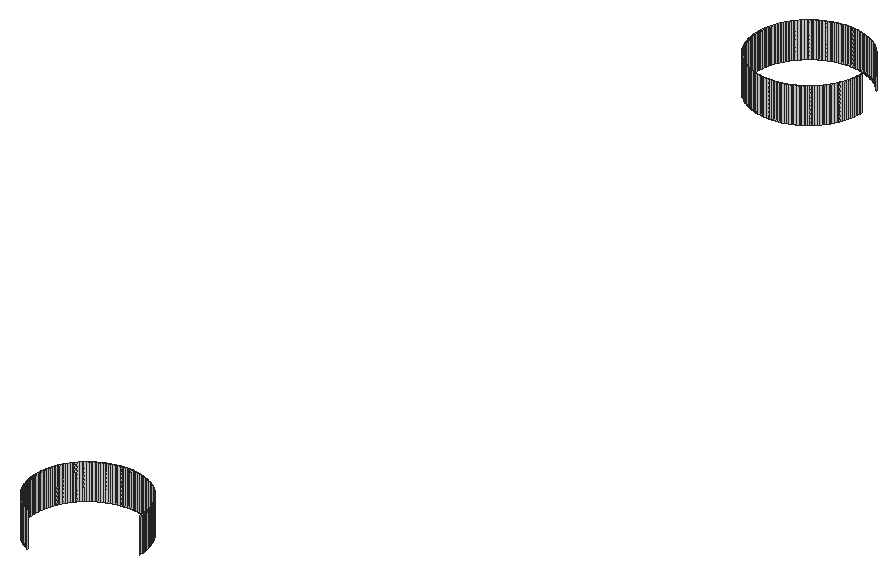
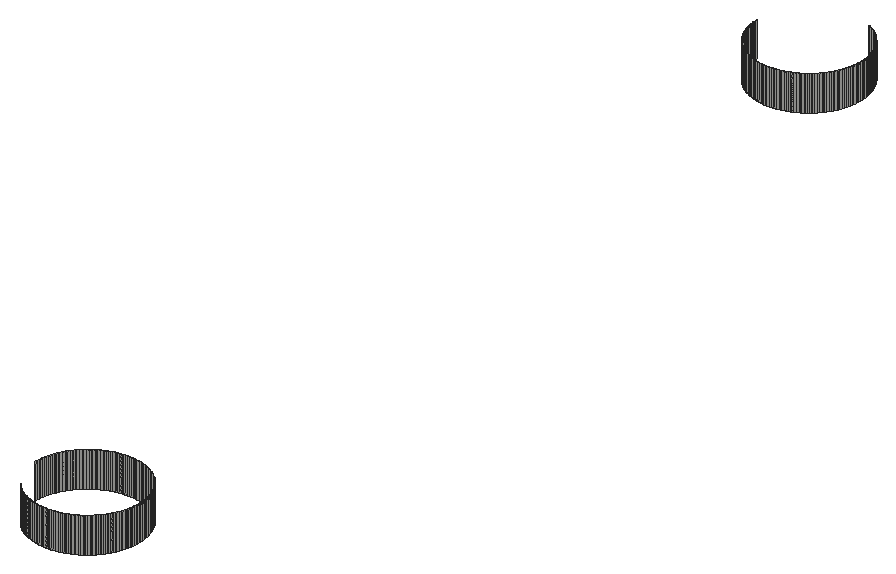
# SketchUp Ruby script. Lengths in inches.
U = 1.inch
M = Sketchup.active_model
def pt(a) = Geom::Point3d.new(a.map { |v| v * U })
def face(e, loops, mat)
  f = e.add_face(loops[0].map { |a| pt(a) })
  loops[1..].each { |l| e.add_face(l.map { |a| pt(a) }).erase! }
  f.material = f.back_material = mat if mat
  f
end
# faces: each face lists its corners as indices into pts; further lists are holes
def faces(e, pts, list, mat = nil) = list.each { |f| face(e, (f[0].is_a?(Array) ? f : [f]).map { |l| l.map { |i| pts[i] } }, mat) }
# xy, xz, yz: faces in a plane at the given z, y or x. An outline is a flat list of corners, or four numbers for a rectangle; further outlines are holes
def ring(l) = l.size == 4 ? [[l[0], l[1]], [l[2], l[1]], [l[2], l[3]], [l[0], l[3]]] : l.each_slice(2).to_a
def flat(e, list, mat, &to3) = list.each { |f| face(e, (f[0].is_a?(Array) ? f : [f]).map { |l| ring(l).map { |u, v| to3.(u, v) } }, mat) }
def xy(e, z, list, mat = nil) = flat(e, list, mat) { |x, y| [x, y, z] }
def xz(e, y, list, mat = nil) = flat(e, list, mat) { |x, z| [x, y, z] }
def yz(e, x, list, mat = nil) = flat(e, list, mat) { |y, z| [x, y, z] }
def lines(e, pts, list) = list.each { |a, b| e.add_line(pt(pts[a]), pt(pts[b])) }
# prism: a flat outline (further loops are holes) pulled along v
def prism(e, loops, v, mat = nil)
  f = face(e, loops, mat); d = Geom::Vector3d.new(v.map { |x| x * U })
  f.pushpull(f.normal.samedirection?(d) ? d.length : -d.length)
end
def box(e, o, s, mat = nil) = prism(e, [[o, [o[0] + s[0], o[1], o[2]], [o[0] + s[0], o[1] + s[1], o[2]], [o[0], o[1] + s[1], o[2]]]], [0, 0, s[2]], mat)
def at(x, y, z, deg = 0) = Geom::Transformation.translation(pt([x, y, z])) * Geom::Transformation.rotation(ORIGIN, Z_AXIS, deg.degrees)
def axes(o, x, y, z) = Geom::Transformation.new([*x, 0, *y, 0, *z, 0, *pt(o).to_a, 1])
def part(name) = M.definitions.add(name)
# library, detail: a bought-in or finely detailed component or shape, given as its bounding box
def library(name, o, s) = part(name).tap { |d| box(d.entities, o, s) }
def detail(e, o, s) = box(e.add_group.entities, o, s)
def put(e, d, t, mat = nil) = e.add_instance(d, t).tap { |i| i.material = mat if mat }
def group(e, t, mat = nil) = e.add_group.tap { |g| g.transformation = t; g.material = mat if mat }.entities
root = M.entities
xz(root,78.5,[[156.34,108,156.42,110],[156.42,108,156.5,110],[156.5,108,156.58,110],[156.58,108,156.66,110]])
xz(root,124,[[156.34,108,156.42,110],[156.42,108,156.5,110],[156.5,108,156.58,110],[156.58,108,156.66,110]])
xz(root,130,[[156.34,108,156.42,110],[156.42,108,156.5,110],[156.5,108,156.58,110],[156.58,108,156.66,110]])
yz(root,153.5,[[75.34,108,75.42,110],[75.42,108,75.5,110],[75.5,108,75.58,110],[75.58,108,75.66,110],[126.84,108,126.92,110],
  [126.92,108,127,110],[127,108,127.08,110],[127.08,108,127.16,110]])
yz(root,159.5,[[75.5,108,75.58,110],[75.58,108,75.66,110],[126.84,108,126.92,110],[126.92,108,127,110]])
p = [[155.21,72.79,108],[155.14,72.83,108],[155.14,72.83,110],[155.21,72.79,110],[155.07,72.86,108],[155.07,72.86,110],
  [155.28,72.76,108],[155.28,72.76,110],[155,72.9,108],[154.93,72.94,108],[154.93,72.94,110],[155,72.9,110],
  [154.87,72.98,108],[154.87,72.98,110],[154.8,73.03,108],[154.74,73.07,108],[154.74,73.07,110],[154.8,73.03,110],
  [154.67,73.12,108],[154.61,73.17,108],[154.61,73.17,110],[154.67,73.12,110],[154.55,73.22,108],[154.49,73.27,108],
  [154.49,73.27,110],[154.55,73.22,110],[154.43,73.32,108],[154.43,73.32,110],[154.38,73.38,108],[154.38,73.38,110],
  [154.32,73.43,108],[154.32,73.43,110],[154.27,73.49,108],[154.27,73.49,110],[154.22,73.55,108],[154.22,73.55,110],
  [154.17,73.61,108],[154.12,73.67,108],[154.12,73.67,110],[154.17,73.61,110],[154.07,73.74,108],[154.03,73.8,108],
  [154.03,73.8,110],[154.07,73.74,110],[153.98,73.87,108],[153.98,73.87,110],[153.94,73.93,108],[153.94,73.93,110],
  [153.9,74,108],[153.9,74,110],[153.86,74.07,108],[153.86,74.07,110],[153.83,74.14,108],[153.83,74.14,110],
  [153.79,74.21,108],[153.79,74.21,110],[153.76,74.28,108],[153.76,74.28,110],[153.73,74.35,108],[153.73,74.35,110],
  [153.7,74.42,108],[153.7,74.42,110],[153.67,74.5,108],[153.67,74.5,110],[153.65,74.57,108],[153.65,74.57,110],
  [153.625,74.65,108],[153.625,74.65,110],[153.6,74.72,108],[153.6,74.72,110],[153.58,74.8,108],[153.58,74.8,110],
  [153.57,74.875,108],[153.57,74.875,110],[153.55,74.95,108],[153.55,74.95,110],[153.54,75.03,108],[153.54,75.03,110],
  [153.53,75.11,108],[153.53,75.11,110],[153.52,75.1875,108],[153.52,75.1875,110],[153.51,75.26,108],[153.51,75.26,110],
  [153.5,75.34,108],[153.5,75.34,110],[153.5,75.66,108],[153.51,75.74,108],[153.51,75.74,110],[153.5,75.66,110],
  [153.52,75.8125,108],[153.52,75.8125,110],[159.48,75.8125,108],[159.49,75.74,108],[159.49,75.74,110],[159.48,75.8125,110],
  [159.5,75.66,108],[159.5,75.66,110],[153.53,75.89,108],[153.53,75.89,110],[159.47,75.89,108],[159.47,75.89,110],
  [153.54,75.97,108],[153.54,75.97,110],[159.46,75.97,108],[159.46,75.97,110],[153.55,76.05,108],[153.55,76.05,110],
  [153.57,76.125,108],[153.57,76.125,110],[159.43,76.125,108],[159.45,76.05,108],[159.45,76.05,110],[159.43,76.125,110],
  [153.58,76.2,108],[153.58,76.2,110],[159.42,76.2,108],[159.42,76.2,110],[153.6,76.28,108],[153.6,76.28,110],
  [159.4,76.28,108],[159.4,76.28,110],[153.625,76.35,108],[153.625,76.35,110],[159.375,76.35,108],[159.375,76.35,110],
  [153.65,76.43,108],[153.65,76.43,110],[153.67,76.5,108],[153.67,76.5,110],[159.33,76.5,108],[159.35,76.43,108],
  [159.35,76.43,110],[159.33,76.5,110],[153.7,76.58,108],[153.7,76.58,110],[159.3,76.58,108],[159.3,76.58,110],
  [153.73,76.65,108],[153.73,76.65,110],[153.76,76.72,108],[153.76,76.72,110],[159.24,76.72,108],[159.27,76.65,108],
  [159.27,76.65,110],[159.24,76.72,110],[153.79,76.79,108],[153.79,76.79,110],[159.21,76.79,108],[159.21,76.79,110],
  [153.83,76.86,108],[153.83,76.86,110],[159.17,76.86,108],[159.17,76.86,110],[153.86,76.93,108],[153.86,76.93,110],
  [153.9,77,108],[153.9,77,110],[159.1,77,108],[159.14,76.93,108],[159.14,76.93,110],[159.1,77,110],
  [153.94,77.07,108],[153.94,77.07,110],[159.06,77.07,108],[159.06,77.07,110],[153.98,77.13,108],[153.98,77.13,110],
  [154.03,77.2,108],[154.03,77.2,110],[158.97,77.2,108],[159.02,77.13,108],[159.02,77.13,110],[158.97,77.2,110],
  [154.07,77.26,108],[154.07,77.26,110],[158.93,77.26,108],[158.93,77.26,110],[154.12,77.33,108],[154.12,77.33,110],
  [154.17,77.39,108],[154.17,77.39,110],[158.83,77.39,108],[158.88,77.33,108],[158.88,77.33,110],[158.83,77.39,110],
  [154.22,77.45,108],[154.22,77.45,110],[154.27,77.51,108],[154.27,77.51,110],[158.73,77.51,108],[158.78,77.45,108],
  [158.78,77.45,110],[158.73,77.51,110],[154.32,77.57,108],[154.32,77.57,110],[158.68,77.57,108],[158.68,77.57,110],
  [154.38,77.62,108],[154.38,77.62,110],[154.43,77.68,108],[154.43,77.68,110],[158.57,77.68,108],[158.62,77.62,108],
  [158.62,77.62,110],[158.57,77.68,110],[154.49,77.73,108],[154.49,77.73,110],[154.55,77.78,108],[154.55,77.78,110],
  [158.45,77.78,108],[158.51,77.73,108],[158.51,77.73,110],[158.45,77.78,110],[154.61,77.83,108],[154.61,77.83,110],
  [154.67,77.88,108],[154.67,77.88,110],[158.33,77.88,108],[158.39,77.83,108],[158.39,77.83,110],[158.33,77.88,110],
  [154.74,77.93,108],[154.74,77.93,110],[154.8,77.97,108],[154.8,77.97,110],[158.2,77.97,108],[158.26,77.93,108],
  [158.26,77.93,110],[158.2,77.97,110],[154.87,78.02,108],[154.87,78.02,110],[154.93,78.06,108],[154.93,78.06,110],
  [158.07,78.06,108],[158.13,78.02,108],[158.13,78.02,110],[158.07,78.06,110],[155,78.1,108],[155,78.1,110],
  [155.07,78.14,108],[155.07,78.14,110],[155.14,78.17,108],[155.14,78.17,110],[157.86,78.17,108],[157.93,78.14,108],
  [157.93,78.14,110],[157.86,78.17,110],[158,78.1,108],[158,78.1,110],[155.21,78.21,108],[155.21,78.21,110],
  [155.28,78.24,108],[155.28,78.24,110],[155.35,78.27,108],[155.35,78.27,110],[157.65,78.27,108],[157.72,78.24,108],
  [157.72,78.24,110],[157.65,78.27,110],[157.79,78.21,108],[157.79,78.21,110],[155.42,78.3,108],[155.42,78.3,110],
  [155.5,78.33,108],[155.5,78.33,110],[155.57,78.35,108],[155.57,78.35,110],[157.43,78.35,108],[157.5,78.33,108],
  [157.5,78.33,110],[157.43,78.35,110],[157.58,78.3,108],[157.58,78.3,110],[155.65,78.375,108],[155.65,78.375,110],
  [155.72,78.4,108],[155.72,78.4,110],[155.8,78.42,108],[155.8,78.42,110],[155.875,78.43,108],[155.875,78.43,110],
  [155.95,78.45,108],[155.95,78.45,110],[156.03,78.46,108],[156.03,78.46,110],[156.97,78.46,108],[157.05,78.45,108],
  [157.05,78.45,110],[156.97,78.46,110],[157.125,78.43,108],[157.125,78.43,110],[157.2,78.42,108],[157.2,78.42,110],
  [157.28,78.4,108],[157.28,78.4,110],[157.35,78.375,108],[157.35,78.375,110],[156.11,78.47,108],[156.11,78.47,110],
  [156.1875,78.48,108],[156.1875,78.48,110],[156.26,78.49,108],[156.26,78.49,110],[156.34,78.5,108],[156.34,78.5,110],
  [156.66,78.5,108],[156.74,78.49,108],[156.74,78.49,110],[156.66,78.5,110],[156.8125,78.48,108],[156.8125,78.48,110],
  [156.89,78.47,108],[156.89,78.47,110],[156.11,124.03,108],[156.03,124.04,108],[156.03,124.04,110],[156.11,124.03,110],
  [155.95,124.05,108],[155.95,124.05,110],[156.1875,124.02,108],[156.1875,124.02,110],[156.26,124.01,108],[156.26,124.01,110],
  [156.34,124,108],[156.34,124,110],[156.8125,124.02,108],[156.74,124.01,108],[156.74,124.01,110],[156.8125,124.02,110],
  [156.66,124,108],[156.66,124,110],[156.89,124.03,108],[156.89,124.03,110],[156.97,124.04,108],[156.97,124.04,110],
  [157.05,124.05,108],[157.05,124.05,110],[155.57,124.15,108],[155.5,124.17,108],[155.5,124.17,110],[155.57,124.15,110],
  [155.72,124.1,108],[155.65,124.125,108],[155.65,124.125,110],[155.72,124.1,110],[155.8,124.08,108],[155.8,124.08,110],
  [155.875,124.07,108],[155.875,124.07,110],[157.125,124.07,108],[157.125,124.07,110],[157.2,124.08,108],[157.2,124.08,110],
  [157.28,124.1,108],[157.28,124.1,110],[157.35,124.125,108],[157.35,124.125,110],[157.5,124.17,108],[157.43,124.15,108],
  [157.43,124.15,110],[157.5,124.17,110],[155.35,124.23,108],[155.28,124.26,108],[155.28,124.26,110],[155.35,124.23,110],
  [155.42,124.2,108],[155.42,124.2,110],[157.58,124.2,108],[157.58,124.2,110],[157.72,124.26,108],[157.65,124.23,108],
  [157.65,124.23,110],[157.72,124.26,110],[155.21,124.29,108],[155.14,124.33,108],[155.14,124.33,110],[155.21,124.29,110],
  [155.07,124.36,108],[155.07,124.36,110],[157.79,124.29,108],[157.79,124.29,110],[157.86,124.33,108],[157.86,124.33,110],
  [157.93,124.36,108],[157.93,124.36,110],[155,124.4,108],[154.93,124.44,108],[154.93,124.44,110],[155,124.4,110],
  [154.87,124.48,108],[154.87,124.48,110],[158,124.4,108],[158,124.4,110],[158.07,124.44,108],[158.07,124.44,110],
  [158.13,124.48,108],[158.13,124.48,110],[154.8,124.53,108],[154.74,124.57,108],[154.74,124.57,110],[154.8,124.53,110],
  [158.2,124.53,108],[158.2,124.53,110],[158.26,124.57,108],[158.26,124.57,110],[154.67,124.62,108],[154.61,124.67,108],
  [154.61,124.67,110],[154.67,124.62,110],[158.39,124.67,108],[158.33,124.62,108],[158.33,124.62,110],[158.39,124.67,110],
  [154.55,124.72,108],[154.49,124.77,108],[154.49,124.77,110],[154.55,124.72,110],[158.51,124.77,108],[158.45,124.72,108],
  [158.45,124.72,110],[158.51,124.77,110],[154.43,124.82,108],[154.43,124.82,110],[154.38,124.88,108],[154.38,124.88,110],
  [158.57,124.82,108],[158.57,124.82,110],[158.62,124.88,108],[158.62,124.88,110],[154.32,124.93,108],[154.32,124.93,110],
  [154.27,124.99,108],[154.27,124.99,110],[158.68,124.93,108],[158.68,124.93,110],[158.73,124.99,108],[158.73,124.99,110],
  [154.22,125.05,108],[154.22,125.05,110],[158.78,125.05,108],[158.78,125.05,110],[154.17,125.11,108],[154.12,125.17,108],
  [154.12,125.17,110],[154.17,125.11,110],[158.88,125.17,108],[158.83,125.11,108],[158.83,125.11,110],[158.88,125.17,110],
  [154.07,125.24,108],[154.03,125.3,108],[154.03,125.3,110],[154.07,125.24,110],[158.97,125.3,108],[158.93,125.24,108],
  [158.93,125.24,110],[158.97,125.3,110],[153.98,125.37,108],[153.98,125.37,110],[159.02,125.37,108],[159.02,125.37,110],
  [153.94,125.43,108],[153.94,125.43,110],[153.9,125.5,108],[153.9,125.5,110],[159.06,125.43,108],[159.06,125.43,110],
  [159.1,125.5,108],[159.1,125.5,110],[153.86,125.57,108],[153.86,125.57,110],[159.14,125.57,108],[159.14,125.57,110],
  [153.83,125.64,108],[153.83,125.64,110],[153.79,125.71,108],[153.79,125.71,110],[159.17,125.64,108],[159.17,125.64,110],
  [159.21,125.71,108],[159.21,125.71,110],[153.76,125.78,108],[153.76,125.78,110],[159.24,125.78,108],[159.24,125.78,110],
  [153.73,125.85,108],[153.73,125.85,110],[159.27,125.85,108],[159.27,125.85,110],[153.7,125.92,108],[153.7,125.92,110],
  [153.67,126,108],[153.67,126,110],[159.33,126,108],[159.3,125.92,108],[159.3,125.92,110],[159.33,126,110],
  [153.65,126.07,108],[153.65,126.07,110],[159.35,126.07,108],[159.35,126.07,110],[153.625,126.15,108],[153.625,126.15,110],
  [153.6,126.22,108],[153.6,126.22,110],[159.4,126.22,108],[159.375,126.15,108],[159.375,126.15,110],[159.4,126.22,110],
  [153.58,126.3,108],[153.58,126.3,110],[159.42,126.3,108],[159.42,126.3,110],[153.57,126.375,108],[153.57,126.375,110],
  [159.43,126.375,108],[159.43,126.375,110],[153.55,126.45,108],[153.55,126.45,110],[159.45,126.45,108],[159.45,126.45,110],
  [153.54,126.53,108],[153.54,126.53,110],[153.53,126.61,108],[153.53,126.61,110],[159.46,126.53,108],[159.46,126.53,110],
  [159.47,126.61,108],[159.47,126.61,110],[153.52,126.6875,108],[153.52,126.6875,110],[159.48,126.6875,108],[159.48,126.6875,110],
  [153.51,126.76,108],[153.51,126.76,110],[159.49,126.76,108],[159.49,126.76,110],[153.5,126.84,108],[153.5,126.84,110],
  [159.5,126.84,108],[159.5,126.84,110],[153.5,127.16,108],[153.51,127.24,108],[153.51,127.24,110],[153.5,127.16,110],
  [153.52,127.3125,108],[153.52,127.3125,110],[153.53,127.39,108],[153.53,127.39,110],[153.54,127.47,108],[153.54,127.47,110],
  [153.55,127.55,108],[153.55,127.55,110],[153.57,127.625,108],[153.57,127.625,110],[153.58,127.7,108],[153.58,127.7,110],
  [153.6,127.78,108],[153.6,127.78,110],[153.625,127.85,108],[153.625,127.85,110],[153.65,127.93,108],[153.65,127.93,110],
  [153.67,128,108],[153.67,128,110],[153.7,128.08,108],[153.7,128.08,110],[153.73,128.15,108],[153.73,128.15,110],
  [153.76,128.22,108],[153.76,128.22,110],[153.79,128.29,108],[153.79,128.29,110],[153.83,128.36,108],[153.83,128.36,110],
  [153.86,128.43,108],[153.86,128.43,110],[153.9,128.5,108],[153.9,128.5,110],[153.94,128.57,108],[153.94,128.57,110],
  [153.98,128.63,108],[153.98,128.63,110],[154.03,128.7,108],[154.03,128.7,110],[154.07,128.76,108],[154.07,128.76,110],
  [154.12,128.83,108],[154.12,128.83,110],[154.17,128.89,108],[154.17,128.89,110],[154.22,128.95,108],[154.22,128.95,110],
  [154.27,129.01,108],[154.27,129.01,110],[158.73,129.01,108],[158.78,128.95,108],[158.78,128.95,110],[158.73,129.01,110],
  [154.32,129.07,108],[154.32,129.07,110],[158.68,129.07,108],[158.68,129.07,110],[154.38,129.12,108],[154.38,129.12,110],
  [154.43,129.18,108],[154.43,129.18,110],[158.57,129.18,108],[158.62,129.12,108],[158.62,129.12,110],[158.57,129.18,110],
  [154.49,129.23,108],[154.49,129.23,110],[154.55,129.28,108],[154.55,129.28,110],[158.45,129.28,108],[158.51,129.23,108],
  [158.51,129.23,110],[158.45,129.28,110],[154.61,129.33,108],[154.61,129.33,110],[154.67,129.38,108],[154.67,129.38,110],
  [158.33,129.38,108],[158.39,129.33,108],[158.39,129.33,110],[158.33,129.38,110],[154.74,129.43,108],[154.74,129.43,110],
  [154.8,129.47,108],[154.8,129.47,110],[158.2,129.47,108],[158.26,129.43,108],[158.26,129.43,110],[158.2,129.47,110],
  [154.87,129.52,108],[154.87,129.52,110],[154.93,129.56,108],[154.93,129.56,110],[158.07,129.56,108],[158.13,129.52,108],
  [158.13,129.52,110],[158.07,129.56,110],[155,129.6,108],[155,129.6,110],[155.07,129.64,108],[155.07,129.64,110],
  [155.14,129.67,108],[155.14,129.67,110],[157.86,129.67,108],[157.93,129.64,108],[157.93,129.64,110],[157.86,129.67,110],
  [158,129.6,108],[158,129.6,110],[155.21,129.71,108],[155.21,129.71,110],[155.28,129.74,108],[155.28,129.74,110],
  [155.35,129.77,108],[155.35,129.77,110],[157.65,129.77,108],[157.72,129.74,108],[157.72,129.74,110],[157.65,129.77,110],
  [157.79,129.71,108],[157.79,129.71,110],[155.42,129.8,108],[155.42,129.8,110],[155.5,129.83,108],[155.5,129.83,110],
  [155.57,129.85,108],[155.57,129.85,110],[157.43,129.85,108],[157.5,129.83,108],[157.5,129.83,110],[157.43,129.85,110],
  [157.58,129.8,108],[157.58,129.8,110],[155.65,129.875,108],[155.65,129.875,110],[155.72,129.9,108],[155.72,129.9,110],
  [155.8,129.92,108],[155.8,129.92,110],[155.875,129.93,108],[155.875,129.93,110],[155.95,129.95,108],[155.95,129.95,110],
  [156.03,129.96,108],[156.03,129.96,110],[156.97,129.96,108],[157.05,129.95,108],[157.05,129.95,110],[156.97,129.96,110],
  [157.125,129.93,108],[157.125,129.93,110],[157.2,129.92,108],[157.2,129.92,110],[157.28,129.9,108],[157.28,129.9,110],
  [157.35,129.875,108],[157.35,129.875,110],[156.11,129.97,108],[156.11,129.97,110],[156.1875,129.98,108],[156.1875,129.98,110],
  [156.26,129.99,108],[156.26,129.99,110],[156.34,130,108],[156.34,130,110],[156.66,130,108],[156.74,129.99,108],
  [156.74,129.99,110],[156.66,130,110],[156.8125,129.98,108],[156.8125,129.98,110],[156.89,129.97,108],[156.89,129.97,110]]
faces(root,p,[[0,1,2,3],[1,4,5,2],[6,0,3,7],[8,9,10,11],[9,12,13,10],[4,8,11,5],[14,15,16,17],[12,14,17,13],
  [18,19,20,21],[15,18,21,16],[22,23,24,25],[19,22,25,20],[23,26,27,24],[26,28,29,27],[28,30,31,29],[30,32,33,31],
  [32,34,35,33],[36,37,38,39],[34,36,39,35],[40,41,42,43],[37,40,43,38],[41,44,45,42],[44,46,47,45],[46,48,49,47],
  [48,50,51,49],[50,52,53,51],[52,54,55,53],[54,56,57,55],[56,58,59,57],[58,60,61,59],[60,62,63,61],[62,64,65,63],
  [64,66,67,65],[66,68,69,67],[68,70,71,69],[70,72,73,71],[72,74,75,73],[74,76,77,75],[76,78,79,77],[78,80,81,79],
  [80,82,83,81],[82,84,85,83],[86,87,88,89],[87,90,91,88],[92,93,94,95],[93,96,97,94],[90,98,99,91],[100,92,95,101],
  [98,102,103,99],[104,100,101,105],[102,106,107,103],[106,108,109,107],[110,111,112,113],[111,104,105,112],[108,114,115,109],[116,110,113,117],
  [114,118,119,115],[120,116,117,121],[118,122,123,119],[124,120,121,125],[122,126,127,123],[126,128,129,127],[130,131,132,133],[131,124,125,132],
  [128,134,135,129],[136,130,133,137],[134,138,139,135],[138,140,141,139],[142,143,144,145],[143,136,137,144],[140,146,147,141],[148,142,145,149],
  [146,150,151,147],[152,148,149,153],[150,154,155,151],[154,156,157,155],[158,159,160,161],[159,152,153,160],[156,162,163,157],[164,158,161,165],
  [162,166,167,163],[166,168,169,167],[170,171,172,173],[171,164,165,172],[168,174,175,169],[176,170,173,177],[174,178,179,175],[178,180,181,179],
  [182,183,184,185],[183,176,177,184],[180,186,187,181],[186,188,189,187],[190,191,192,193],[191,182,185,192],[188,194,195,189],[196,190,193,197],
  [194,198,199,195],[198,200,201,199],[202,203,204,205],[203,196,197,204],[200,206,207,201],[206,208,209,207],[210,211,212,213],[211,202,205,212],
  [208,214,215,209],[214,216,217,215],[218,219,220,221],[219,210,213,220],[216,222,223,217],[222,224,225,223],[226,227,228,229],[227,218,221,228],
  [224,230,231,225],[230,232,233,231],[234,235,236,237],[235,226,229,236],[232,238,239,233],[238,240,241,239],[240,242,243,241],[244,245,246,247],
  [245,248,249,246],[248,234,237,249],[242,250,251,243],[250,252,253,251],[252,254,255,253],[256,257,258,259],[257,260,261,258],[260,244,247,261],
  [254,262,263,255],[262,264,265,263],[264,266,267,265],[268,269,270,271],[269,272,273,270],[272,256,259,273],[266,274,275,267],[274,276,277,275],
  [276,278,279,277],[278,280,281,279],[280,282,283,281],[282,284,285,283],[286,287,288,289],[287,290,291,288],[290,292,293,291],[292,294,295,293],
  [294,296,297,295],[296,268,271,297],[284,298,299,285],[298,300,301,299],[300,302,303,301],[302,304,305,303],[306,307,308,309],[307,310,311,308],
  [310,312,313,311],[312,286,289,313],[314,315,316,317],[315,318,319,316],[320,314,317,321],[322,320,321,323],[324,322,323,325],[326,327,328,329],
  [327,330,331,328],[332,326,329,333],[334,332,333,335],[336,334,335,337],[338,339,340,341],[342,343,344,345],[343,338,341,344],[346,342,345,347],
  [348,346,347,349],[318,348,349,319],[350,336,337,351],[352,350,351,353],[354,352,353,355],[356,354,355,357],[358,359,360,361],[359,356,357,360],
  [362,363,364,365],[339,366,367,340],[366,362,365,367],[368,358,361,369],[370,371,372,373],[371,368,369,372],[374,375,376,377],[375,378,379,376],
  [363,374,377,364],[380,370,373,381],[382,380,381,383],[384,382,383,385],[386,387,388,389],[387,390,391,388],[378,386,389,379],[392,384,385,393],
  [394,392,393,395],[396,394,395,397],[398,399,400,401],[390,398,401,391],[402,396,397,403],[404,402,403,405],[406,407,408,409],[399,406,409,400],
  [410,411,412,413],[411,404,405,412],[414,415,416,417],[407,414,417,408],[418,419,420,421],[419,410,413,420],[415,422,423,416],[422,424,425,423],
  [426,418,421,427],[428,426,427,429],[424,430,431,425],[430,432,433,431],[434,428,429,435],[436,434,435,437],[432,438,439,433],[440,436,437,441],
  [442,443,444,445],[438,442,445,439],[446,447,448,449],[447,440,441,448],[450,451,452,453],[443,450,453,444],[454,455,456,457],[455,446,449,456],
  [451,458,459,452],[460,454,457,461],[458,462,463,459],[462,464,465,463],[466,460,461,467],[468,466,467,469],[464,470,471,465],[472,468,469,473],
  [470,474,475,471],[474,476,477,475],[478,472,473,479],[480,478,479,481],[476,482,483,477],[484,480,481,485],[482,486,487,483],[488,484,485,489],
  [486,490,491,487],[490,492,493,491],[494,495,496,497],[495,488,489,496],[492,498,499,493],[500,494,497,501],[498,502,503,499],[502,504,505,503],
  [506,507,508,509],[507,500,501,508],[504,510,511,505],[512,506,509,513],[510,514,515,511],[516,512,513,517],[514,518,519,515],[520,516,517,521],
  [518,522,523,519],[522,524,525,523],[526,520,521,527],[528,526,527,529],[524,530,531,525],[532,528,529,533],[530,534,535,531],[536,532,533,537],
  [534,538,539,535],[540,536,537,541],[542,543,544,545],[543,546,547,544],[546,548,549,547],[548,550,551,549],[550,552,553,551],[552,554,555,553],
  [554,556,557,555],[556,558,559,557],[558,560,561,559],[560,562,563,561],[562,564,565,563],[564,566,567,565],[566,568,569,567],[568,570,571,569],
  [570,572,573,571],[572,574,575,573],[574,576,577,575],[576,578,579,577],[578,580,581,579],[580,582,583,581],[582,584,585,583],[584,586,587,585],
  [586,588,589,587],[588,590,591,589],[590,592,593,591],[592,594,595,593],[596,597,598,599],[594,600,601,595],[602,596,599,603],[600,604,605,601],
  [604,606,607,605],[608,609,610,611],[609,602,603,610],[606,612,613,607],[612,614,615,613],[616,617,618,619],[617,608,611,618],[614,620,621,615],
  [620,622,623,621],[624,625,626,627],[625,616,619,626],[622,628,629,623],[628,630,631,629],[632,633,634,635],[633,624,627,634],[630,636,637,631],
  [636,638,639,637],[640,641,642,643],[641,632,635,642],[638,644,645,639],[644,646,647,645],[646,648,649,647],[650,651,652,653],[651,654,655,652],
  [654,640,643,655],[648,656,657,649],[656,658,659,657],[658,660,661,659],[662,663,664,665],[663,666,667,664],[666,650,653,667],[660,668,669,661],
  [668,670,671,669],[670,672,673,671],[674,675,676,677],[675,678,679,676],[678,662,665,679],[672,680,681,673],[680,682,683,681],[682,684,685,683],
  [684,686,687,685],[686,688,689,687],[688,690,691,689],[692,693,694,695],[693,696,697,694],[696,698,699,697],[698,700,701,699],[700,702,703,701],
  [702,674,677,703],[690,704,705,691],[704,706,707,705],[706,708,709,707],[708,710,711,709],[712,713,714,715],[713,716,717,714],[716,718,719,717],
  [718,692,695,719]])
